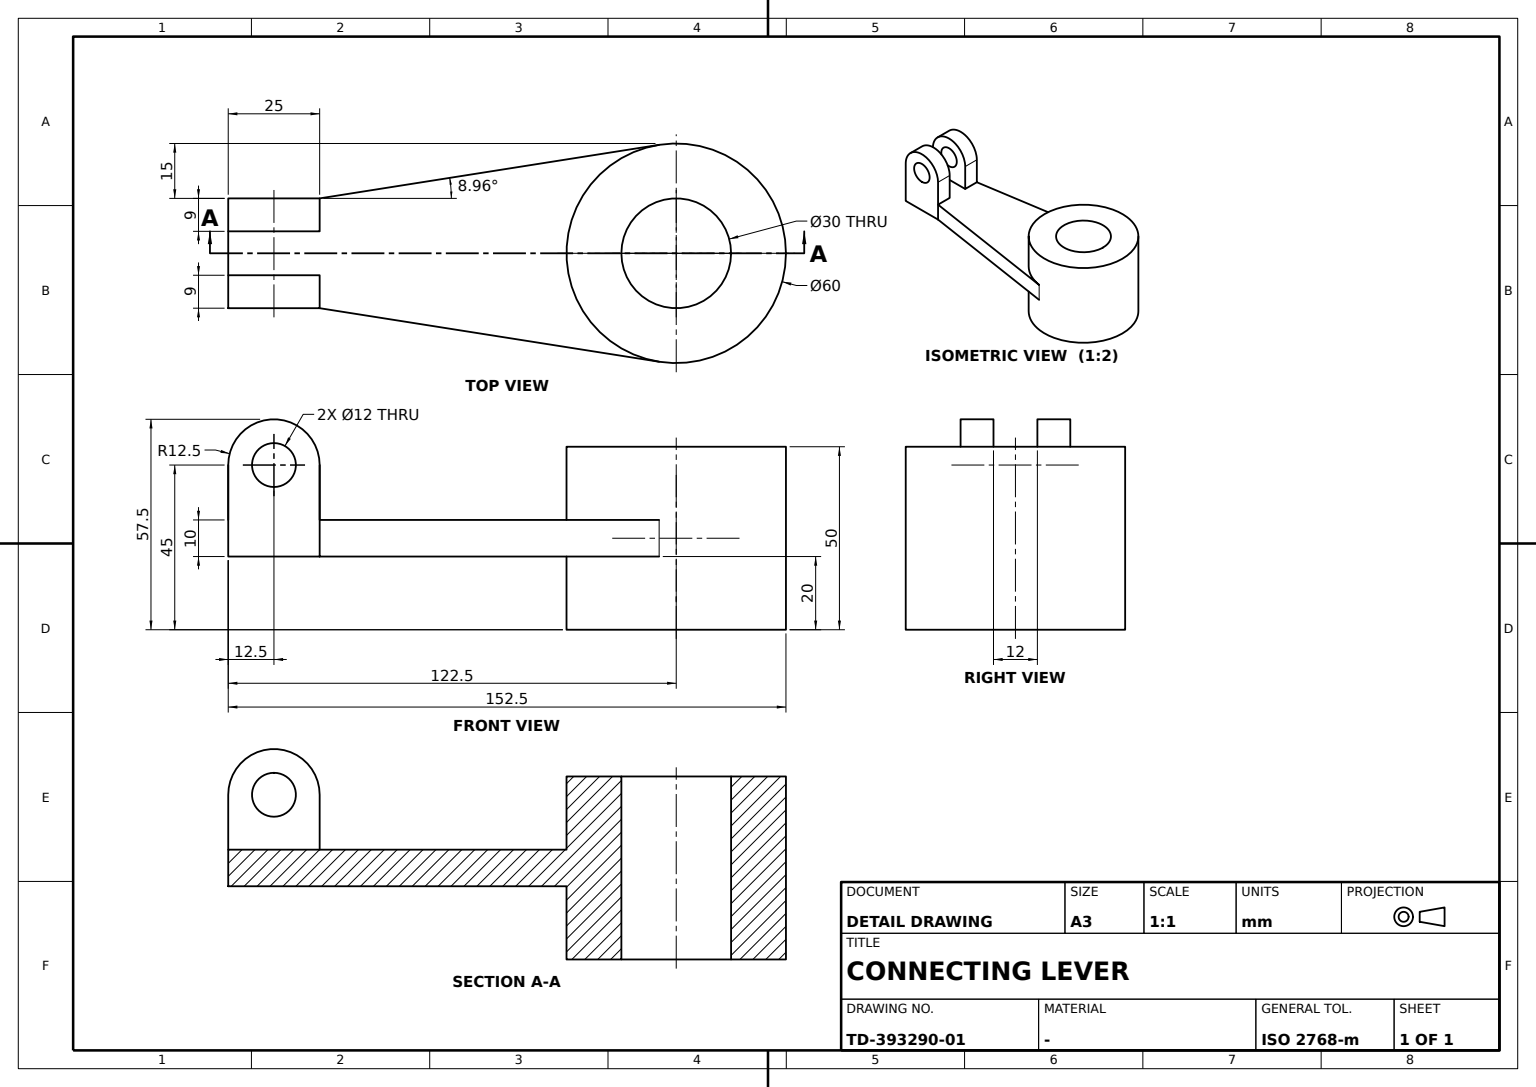
ISO-10303-21;
HEADER;
FILE_DESCRIPTION((''),'2;1');
FILE_NAME('','',(''),(''),'','','');
FILE_SCHEMA(('AUTOMOTIVE_DESIGN'));
ENDSEC;
DATA;
#1=APPLICATION_CONTEXT('');
#2=PRODUCT_CONTEXT('',#1,'mechanical');
#3=PRODUCT('','','',(#2));
#4=PRODUCT_DEFINITION_FORMATION('','',#3);
#5=PRODUCT_DEFINITION_CONTEXT('',#1,'design');
#6=PRODUCT_DEFINITION('','',#4,#5);
#7=PRODUCT_DEFINITION_SHAPE('','',#6);
#8=(LENGTH_UNIT()NAMED_UNIT(*)SI_UNIT(.MILLI.,.METRE.));
#9=(NAMED_UNIT(*)PLANE_ANGLE_UNIT()SI_UNIT($,.RADIAN.));
#10=(NAMED_UNIT(*)SI_UNIT($,.STERADIAN.)SOLID_ANGLE_UNIT());
#11=UNCERTAINTY_MEASURE_WITH_UNIT(LENGTH_MEASURE(0.005),#8,'distance_accuracy_value','');
#12=(GEOMETRIC_REPRESENTATION_CONTEXT(3)GLOBAL_UNCERTAINTY_ASSIGNED_CONTEXT((#11))GLOBAL_UNIT_ASSIGNED_CONTEXT((#8,#9,#10))REPRESENTATION_CONTEXT('',''));
#13=CARTESIAN_POINT('',(-122.5,-6.,20.));
#14=VERTEX_POINT('',#13);
#15=CARTESIAN_POINT('',(-97.5,-6.,20.));
#16=VERTEX_POINT('',#15);
#17=CARTESIAN_POINT('',(-110.,-6.,20.));
#18=DIRECTION('',(0.,1.,0.));
#19=DIRECTION('',(0.,0.,1.));
#20=AXIS2_PLACEMENT_3D('',#17,#18,#19);
#21=CIRCLE('',#20,12.5);
#22=EDGE_CURVE('',#14,#16,#21,.T.);
#23=ORIENTED_EDGE('',*,*,#22,.F.);
#24=CARTESIAN_POINT('',(-122.5,-15.,20.));
#25=VERTEX_POINT('',#24);
#26=CARTESIAN_POINT('',(-122.5,10.5,20.));
#27=VECTOR('',#18,1000.);
#28=LINE('',#26,#27);
#29=EDGE_CURVE('',#25,#14,#28,.T.);
#30=ORIENTED_EDGE('',*,*,#29,.F.);
#31=CARTESIAN_POINT('',(-97.5,-15.,20.));
#32=VERTEX_POINT('',#31);
#33=CARTESIAN_POINT('',(-110.,-15.,20.));
#34=DIRECTION('',(0.,-1.,0.));
#35=DIRECTION('',(0.,0.,-1.));
#36=AXIS2_PLACEMENT_3D('',#33,#34,#35);
#37=CIRCLE('',#36,12.5);
#38=EDGE_CURVE('',#25,#32,#37,.F.);
#39=ORIENTED_EDGE('',*,*,#38,.T.);
#40=CARTESIAN_POINT('',(-97.5,10.5,20.));
#41=LINE('',#40,#27);
#42=EDGE_CURVE('',#32,#16,#41,.T.);
#43=ORIENTED_EDGE('',*,*,#42,.T.);
#44=EDGE_LOOP('',(#23,#30,#39,#43));
#45=FACE_BOUND('',#44,.T.);
#46=CARTESIAN_POINT('',(-110.,10.5,20.));
#47=DIRECTION('',(-1.,0.,0.));
#48=AXIS2_PLACEMENT_3D('',#46,#18,#47);
#49=CYLINDRICAL_SURFACE('',#48,12.5);
#50=ADVANCED_FACE('',(#45),#49,.T.);
#51=CARTESIAN_POINT('',(-110.,15.,26.));
#52=VERTEX_POINT('',#51);
#53=CARTESIAN_POINT('',(-110.,15.,20.));
#54=AXIS2_PLACEMENT_3D('',#53,#18,#19);
#55=CIRCLE('',#54,6.);
#56=EDGE_CURVE('',#52,#52,#55,.T.);
#57=ORIENTED_EDGE('',*,*,#56,.T.);
#58=EDGE_LOOP('',(#57));
#59=FACE_BOUND('',#58,.T.);
#60=CARTESIAN_POINT('',(-110.,6.,26.));
#61=VERTEX_POINT('',#60);
#62=CARTESIAN_POINT('',(-110.,6.,20.));
#63=AXIS2_PLACEMENT_3D('',#62,#18,#19);
#64=CIRCLE('',#63,6.);
#65=EDGE_CURVE('',#61,#61,#64,.T.);
#66=ORIENTED_EDGE('',*,*,#65,.F.);
#67=EDGE_LOOP('',(#66));
#68=FACE_BOUND('',#67,.T.);
#69=CYLINDRICAL_SURFACE('',#48,6.);
#70=ADVANCED_FACE('',(#59,#68),#69,.F.);
#71=ORIENTED_EDGE('',*,*,#56,.F.);
#72=EDGE_LOOP('',(#71));
#73=FACE_BOUND('',#72,.T.);
#74=CARTESIAN_POINT('',(-97.5,15.,20.));
#75=VERTEX_POINT('',#74);
#76=CARTESIAN_POINT('',(-97.5,15.,5.));
#77=VERTEX_POINT('',#76);
#78=VECTOR('',#35,1000.);
#79=LINE('',#74,#78);
#80=EDGE_CURVE('',#75,#77,#79,.T.);
#81=ORIENTED_EDGE('',*,*,#80,.T.);
#82=CARTESIAN_POINT('',(-97.5,15.,-5.));
#83=VERTEX_POINT('',#82);
#84=CARTESIAN_POINT('',(-97.5,15.,0.));
#85=VECTOR('',#19,1000.);
#86=LINE('',#84,#85);
#87=EDGE_CURVE('',#83,#77,#86,.T.);
#88=ORIENTED_EDGE('',*,*,#87,.F.);
#89=CARTESIAN_POINT('',(-122.5,15.,-5.));
#90=VERTEX_POINT('',#89);
#91=CARTESIAN_POINT('',(0.,15.,-5.));
#92=VECTOR('',#47,1000.);
#93=LINE('',#91,#92);
#94=EDGE_CURVE('',#83,#90,#93,.T.);
#95=ORIENTED_EDGE('',*,*,#94,.T.);
#96=CARTESIAN_POINT('',(-122.5,15.,20.));
#97=VERTEX_POINT('',#96);
#98=CARTESIAN_POINT('',(-122.5,15.,0.));
#99=LINE('',#98,#85);
#100=EDGE_CURVE('',#90,#97,#99,.T.);
#101=ORIENTED_EDGE('',*,*,#100,.T.);
#102=CIRCLE('',#54,12.5);
#103=EDGE_CURVE('',#97,#75,#102,.T.);
#104=ORIENTED_EDGE('',*,*,#103,.T.);
#105=EDGE_LOOP('',(#81,#88,#95,#101,#104));
#106=FACE_BOUND('',#105,.T.);
#107=AXIS2_PLACEMENT_3D('',#84,#18,#47);
#108=PLANE('',#107);
#109=ADVANCED_FACE('',(#73,#106),#108,.T.);
#110=CARTESIAN_POINT('',(-4.671689,-29.634023,5.));
#111=VERTEX_POINT('',#110);
#112=CARTESIAN_POINT('',(-97.5,-15.,5.));
#113=VERTEX_POINT('',#112);
#114=DIRECTION('',(-0.987800769,0.155722959,0.));
#115=VECTOR('',#114,1000.);
#116=LINE('',#110,#115);
#117=EDGE_CURVE('',#111,#113,#116,.T.);
#118=ORIENTED_EDGE('',*,*,#117,.T.);
#119=CARTESIAN_POINT('',(-97.5,-15.,-5.));
#120=VERTEX_POINT('',#119);
#121=CARTESIAN_POINT('',(-97.5,-15.,0.));
#122=LINE('',#121,#85);
#123=EDGE_CURVE('',#120,#113,#122,.T.);
#124=ORIENTED_EDGE('',*,*,#123,.F.);
#125=CARTESIAN_POINT('',(-4.671689,-29.634023,-5.));
#126=VERTEX_POINT('',#125);
#127=LINE('',#125,#115);
#128=EDGE_CURVE('',#126,#120,#127,.T.);
#129=ORIENTED_EDGE('',*,*,#128,.F.);
#130=CARTESIAN_POINT('',(-4.671689,-29.634023,0.));
#131=LINE('',#130,#85);
#132=EDGE_CURVE('',#126,#111,#131,.T.);
#133=ORIENTED_EDGE('',*,*,#132,.T.);
#134=EDGE_LOOP('',(#118,#124,#129,#133));
#135=FACE_BOUND('',#134,.T.);
#136=DIRECTION('',(0.155722959,0.987800769,0.));
#137=AXIS2_PLACEMENT_3D('',#130,#136,#114);
#138=PLANE('',#137);
#139=ADVANCED_FACE('',(#135),#138,.F.);
#140=ORIENTED_EDGE('',*,*,#80,.F.);
#141=CARTESIAN_POINT('',(-97.5,6.,20.));
#142=VERTEX_POINT('',#141);
#143=EDGE_CURVE('',#75,#142,#41,.F.);
#144=ORIENTED_EDGE('',*,*,#143,.T.);
#145=CARTESIAN_POINT('',(-97.5,6.,5.));
#146=VERTEX_POINT('',#145);
#147=LINE('',#141,#78);
#148=EDGE_CURVE('',#142,#146,#147,.T.);
#149=ORIENTED_EDGE('',*,*,#148,.T.);
#150=CARTESIAN_POINT('',(-97.5,0.,5.));
#151=VECTOR('',#34,1000.);
#152=LINE('',#150,#151);
#153=EDGE_CURVE('',#77,#146,#152,.T.);
#154=ORIENTED_EDGE('',*,*,#153,.F.);
#155=EDGE_LOOP('',(#140,#144,#149,#154));
#156=FACE_BOUND('',#155,.T.);
#157=AXIS2_PLACEMENT_3D('',#74,#47,#35);
#158=PLANE('',#157);
#159=ADVANCED_FACE('',(#156),#158,.F.);
#160=CARTESIAN_POINT('',(-97.5,-6.,5.));
#161=VERTEX_POINT('',#160);
#162=LINE('',#15,#78);
#163=EDGE_CURVE('',#16,#161,#162,.T.);
#164=ORIENTED_EDGE('',*,*,#163,.T.);
#165=CARTESIAN_POINT('',(-122.5,-6.,5.));
#166=VERTEX_POINT('',#165);
#167=CARTESIAN_POINT('',(0.,-6.,5.));
#168=LINE('',#167,#92);
#169=EDGE_CURVE('',#161,#166,#168,.T.);
#170=ORIENTED_EDGE('',*,*,#169,.T.);
#171=CARTESIAN_POINT('',(-122.5,-6.,0.));
#172=LINE('',#171,#85);
#173=EDGE_CURVE('',#166,#14,#172,.T.);
#174=ORIENTED_EDGE('',*,*,#173,.T.);
#175=ORIENTED_EDGE('',*,*,#22,.T.);
#176=EDGE_LOOP('',(#164,#170,#174,#175));
#177=FACE_BOUND('',#176,.T.);
#178=CARTESIAN_POINT('',(-110.,-6.,26.));
#179=VERTEX_POINT('',#178);
#180=CIRCLE('',#20,6.);
#181=EDGE_CURVE('',#179,#179,#180,.T.);
#182=ORIENTED_EDGE('',*,*,#181,.F.);
#183=EDGE_LOOP('',(#182));
#184=FACE_BOUND('',#183,.T.);
#185=CARTESIAN_POINT('',(0.,-6.,0.));
#186=AXIS2_PLACEMENT_3D('',#185,#18,#47);
#187=PLANE('',#186);
#188=ADVANCED_FACE('',(#177,#184),#187,.T.);
#189=CARTESIAN_POINT('',(15.,0.,-25.));
#190=VERTEX_POINT('',#189);
#191=CARTESIAN_POINT('',(0.,0.,-25.));
#192=DIRECTION('',(1.,0.,0.));
#193=AXIS2_PLACEMENT_3D('',#191,#19,#192);
#194=CIRCLE('',#193,15.);
#195=EDGE_CURVE('',#190,#190,#194,.T.);
#196=ORIENTED_EDGE('',*,*,#195,.T.);
#197=EDGE_LOOP('',(#196));
#198=FACE_BOUND('',#197,.T.);
#199=CARTESIAN_POINT('',(30.,0.,-25.));
#200=VERTEX_POINT('',#199);
#201=CIRCLE('',#193,30.);
#202=EDGE_CURVE('',#200,#200,#201,.T.);
#203=ORIENTED_EDGE('',*,*,#202,.F.);
#204=EDGE_LOOP('',(#203));
#205=FACE_BOUND('',#204,.T.);
#206=PLANE('',#193);
#207=ADVANCED_FACE('',(#198,#205),#206,.F.);
#208=CARTESIAN_POINT('',(-4.671689,29.634023,5.));
#209=VERTEX_POINT('',#208);
#210=DIRECTION('',(-0.987800769,-0.155722959,0.));
#211=VECTOR('',#210,1000.);
#212=LINE('',#208,#211);
#213=EDGE_CURVE('',#209,#77,#212,.T.);
#214=ORIENTED_EDGE('',*,*,#213,.T.);
#215=ORIENTED_EDGE('',*,*,#153,.T.);
#216=CARTESIAN_POINT('',(-122.5,6.,5.));
#217=VERTEX_POINT('',#216);
#218=CARTESIAN_POINT('',(0.,6.,5.));
#219=LINE('',#218,#92);
#220=EDGE_CURVE('',#146,#217,#219,.T.);
#221=ORIENTED_EDGE('',*,*,#220,.T.);
#222=CARTESIAN_POINT('',(-122.5,0.,5.));
#223=LINE('',#222,#151);
#224=EDGE_CURVE('',#217,#166,#223,.T.);
#225=ORIENTED_EDGE('',*,*,#224,.T.);
#226=ORIENTED_EDGE('',*,*,#169,.F.);
#227=LINE('',#76,#27);
#228=EDGE_CURVE('',#113,#161,#227,.T.);
#229=ORIENTED_EDGE('',*,*,#228,.F.);
#230=ORIENTED_EDGE('',*,*,#117,.F.);
#231=CARTESIAN_POINT('',(0.,0.,5.));
#232=AXIS2_PLACEMENT_3D('',#231,#19,#192);
#233=CIRCLE('',#232,30.);
#234=EDGE_CURVE('',#209,#111,#233,.T.);
#235=ORIENTED_EDGE('',*,*,#234,.F.);
#236=EDGE_LOOP('',(#214,#215,#221,#225,#226,#229,#230,#235));
#237=FACE_BOUND('',#236,.T.);
#238=PLANE('',#232);
#239=ADVANCED_FACE('',(#237),#238,.T.);
#240=ORIENTED_EDGE('',*,*,#195,.F.);
#241=EDGE_LOOP('',(#240));
#242=FACE_BOUND('',#241,.T.);
#243=CARTESIAN_POINT('',(15.,0.,25.));
#244=VERTEX_POINT('',#243);
#245=CARTESIAN_POINT('',(0.,0.,25.));
#246=AXIS2_PLACEMENT_3D('',#245,#19,#192);
#247=CIRCLE('',#246,15.);
#248=EDGE_CURVE('',#244,#244,#247,.T.);
#249=ORIENTED_EDGE('',*,*,#248,.T.);
#250=EDGE_LOOP('',(#249));
#251=FACE_BOUND('',#250,.T.);
#252=CARTESIAN_POINT('',(0.,0.,0.));
#253=AXIS2_PLACEMENT_3D('',#252,#19,#192);
#254=CYLINDRICAL_SURFACE('',#253,15.);
#255=ADVANCED_FACE('',(#242,#251),#254,.F.);
#256=ORIENTED_EDGE('',*,*,#173,.F.);
#257=ORIENTED_EDGE('',*,*,#224,.F.);
#258=CARTESIAN_POINT('',(-122.5,6.,20.));
#259=VERTEX_POINT('',#258);
#260=CARTESIAN_POINT('',(-122.5,6.,0.));
#261=LINE('',#260,#85);
#262=EDGE_CURVE('',#217,#259,#261,.T.);
#263=ORIENTED_EDGE('',*,*,#262,.T.);
#264=EDGE_CURVE('',#97,#259,#28,.F.);
#265=ORIENTED_EDGE('',*,*,#264,.F.);
#266=ORIENTED_EDGE('',*,*,#100,.F.);
#267=CARTESIAN_POINT('',(-122.5,-15.,-5.));
#268=VERTEX_POINT('',#267);
#269=CARTESIAN_POINT('',(-122.5,0.,-5.));
#270=LINE('',#269,#151);
#271=EDGE_CURVE('',#90,#268,#270,.T.);
#272=ORIENTED_EDGE('',*,*,#271,.T.);
#273=CARTESIAN_POINT('',(-122.5,-15.,0.));
#274=LINE('',#273,#85);
#275=EDGE_CURVE('',#268,#25,#274,.T.);
#276=ORIENTED_EDGE('',*,*,#275,.T.);
#277=ORIENTED_EDGE('',*,*,#29,.T.);
#278=EDGE_LOOP('',(#256,#257,#263,#265,#266,#272,#276,#277));
#279=FACE_BOUND('',#278,.T.);
#280=AXIS2_PLACEMENT_3D('',#98,#47,#34);
#281=PLANE('',#280);
#282=ADVANCED_FACE('',(#279),#281,.T.);
#283=ORIENTED_EDGE('',*,*,#271,.F.);
#284=ORIENTED_EDGE('',*,*,#94,.F.);
#285=CARTESIAN_POINT('',(-4.671689,29.634023,-5.));
#286=VERTEX_POINT('',#285);
#287=LINE('',#285,#211);
#288=EDGE_CURVE('',#286,#83,#287,.T.);
#289=ORIENTED_EDGE('',*,*,#288,.F.);
#290=CARTESIAN_POINT('',(0.,0.,-5.));
#291=AXIS2_PLACEMENT_3D('',#290,#19,#192);
#292=CIRCLE('',#291,30.);
#293=EDGE_CURVE('',#286,#126,#292,.T.);
#294=ORIENTED_EDGE('',*,*,#293,.T.);
#295=ORIENTED_EDGE('',*,*,#128,.T.);
#296=CARTESIAN_POINT('',(0.,-15.,-5.));
#297=VECTOR('',#192,1000.);
#298=LINE('',#296,#297);
#299=EDGE_CURVE('',#268,#120,#298,.T.);
#300=ORIENTED_EDGE('',*,*,#299,.F.);
#301=EDGE_LOOP('',(#283,#284,#289,#294,#295,#300));
#302=FACE_BOUND('',#301,.T.);
#303=PLANE('',#291);
#304=ADVANCED_FACE('',(#302),#303,.F.);
#305=ORIENTED_EDGE('',*,*,#65,.T.);
#306=EDGE_LOOP('',(#305));
#307=FACE_BOUND('',#306,.T.);
#308=ORIENTED_EDGE('',*,*,#262,.F.);
#309=ORIENTED_EDGE('',*,*,#220,.F.);
#310=ORIENTED_EDGE('',*,*,#148,.F.);
#311=CIRCLE('',#63,12.5);
#312=EDGE_CURVE('',#259,#142,#311,.T.);
#313=ORIENTED_EDGE('',*,*,#312,.F.);
#314=EDGE_LOOP('',(#308,#309,#310,#313));
#315=FACE_BOUND('',#314,.T.);
#316=CARTESIAN_POINT('',(0.,6.,0.));
#317=AXIS2_PLACEMENT_3D('',#316,#18,#47);
#318=PLANE('',#317);
#319=ADVANCED_FACE('',(#307,#315),#318,.F.);
#320=CARTESIAN_POINT('',(30.,0.,25.));
#321=VERTEX_POINT('',#320);
#322=CIRCLE('',#246,30.);
#323=EDGE_CURVE('',#321,#321,#322,.T.);
#324=ORIENTED_EDGE('',*,*,#323,.F.);
#325=EDGE_LOOP('',(#324));
#326=FACE_BOUND('',#325,.T.);
#327=ORIENTED_EDGE('',*,*,#202,.T.);
#328=EDGE_LOOP('',(#327));
#329=FACE_BOUND('',#328,.T.);
#330=ORIENTED_EDGE('',*,*,#293,.F.);
#331=CARTESIAN_POINT('',(-4.671689,29.634023,0.));
#332=LINE('',#331,#85);
#333=EDGE_CURVE('',#286,#209,#332,.T.);
#334=ORIENTED_EDGE('',*,*,#333,.T.);
#335=ORIENTED_EDGE('',*,*,#234,.T.);
#336=ORIENTED_EDGE('',*,*,#132,.F.);
#337=EDGE_LOOP('',(#330,#334,#335,#336));
#338=FACE_BOUND('',#337,.T.);
#339=CYLINDRICAL_SURFACE('',#253,30.);
#340=ADVANCED_FACE('',(#326,#329,#338),#339,.T.);
#341=ORIENTED_EDGE('',*,*,#288,.T.);
#342=ORIENTED_EDGE('',*,*,#87,.T.);
#343=ORIENTED_EDGE('',*,*,#213,.F.);
#344=ORIENTED_EDGE('',*,*,#333,.F.);
#345=EDGE_LOOP('',(#341,#342,#343,#344));
#346=FACE_BOUND('',#345,.T.);
#347=DIRECTION('',(-0.155722959,0.987800769,0.));
#348=AXIS2_PLACEMENT_3D('',#331,#347,#210);
#349=PLANE('',#348);
#350=ADVANCED_FACE('',(#346),#349,.T.);
#351=ORIENTED_EDGE('',*,*,#264,.T.);
#352=ORIENTED_EDGE('',*,*,#312,.T.);
#353=ORIENTED_EDGE('',*,*,#143,.F.);
#354=ORIENTED_EDGE('',*,*,#103,.F.);
#355=EDGE_LOOP('',(#351,#352,#353,#354));
#356=FACE_BOUND('',#355,.T.);
#357=ADVANCED_FACE('',(#356),#49,.T.);
#358=ORIENTED_EDGE('',*,*,#181,.T.);
#359=EDGE_LOOP('',(#358));
#360=FACE_BOUND('',#359,.T.);
#361=CARTESIAN_POINT('',(-110.,-15.,14.));
#362=VERTEX_POINT('',#361);
#363=CIRCLE('',#36,6.);
#364=EDGE_CURVE('',#362,#362,#363,.F.);
#365=ORIENTED_EDGE('',*,*,#364,.F.);
#366=EDGE_LOOP('',(#365));
#367=FACE_BOUND('',#366,.T.);
#368=ADVANCED_FACE('',(#360,#367),#69,.F.);
#369=ORIENTED_EDGE('',*,*,#248,.F.);
#370=EDGE_LOOP('',(#369));
#371=FACE_BOUND('',#370,.T.);
#372=ORIENTED_EDGE('',*,*,#323,.T.);
#373=EDGE_LOOP('',(#372));
#374=FACE_BOUND('',#373,.T.);
#375=PLANE('',#246);
#376=ADVANCED_FACE('',(#371,#374),#375,.T.);
#377=ORIENTED_EDGE('',*,*,#228,.T.);
#378=ORIENTED_EDGE('',*,*,#163,.F.);
#379=ORIENTED_EDGE('',*,*,#42,.F.);
#380=LINE('',#121,#78);
#381=EDGE_CURVE('',#32,#113,#380,.T.);
#382=ORIENTED_EDGE('',*,*,#381,.T.);
#383=EDGE_LOOP('',(#377,#378,#379,#382));
#384=FACE_BOUND('',#383,.T.);
#385=ADVANCED_FACE('',(#384),#158,.F.);
#386=ORIENTED_EDGE('',*,*,#381,.F.);
#387=ORIENTED_EDGE('',*,*,#38,.F.);
#388=ORIENTED_EDGE('',*,*,#275,.F.);
#389=ORIENTED_EDGE('',*,*,#299,.T.);
#390=ORIENTED_EDGE('',*,*,#123,.T.);
#391=EDGE_LOOP('',(#386,#387,#388,#389,#390));
#392=FACE_BOUND('',#391,.T.);
#393=ORIENTED_EDGE('',*,*,#364,.T.);
#394=EDGE_LOOP('',(#393));
#395=FACE_BOUND('',#394,.T.);
#396=AXIS2_PLACEMENT_3D('',#273,#34,#192);
#397=PLANE('',#396);
#398=ADVANCED_FACE('',(#392,#395),#397,.T.);
#399=CLOSED_SHELL('',(#50,#70,#109,#139,#159,#188,#207,#239,#255,#282,#304,#319,#340,#350,#357,#368,#376,#385,#398));
#400=MANIFOLD_SOLID_BREP('',#399);
#401=ADVANCED_BREP_SHAPE_REPRESENTATION('',(#400),#12);
#402=SHAPE_DEFINITION_REPRESENTATION(#7,#401);
ENDSEC;
END-ISO-10303-21;
